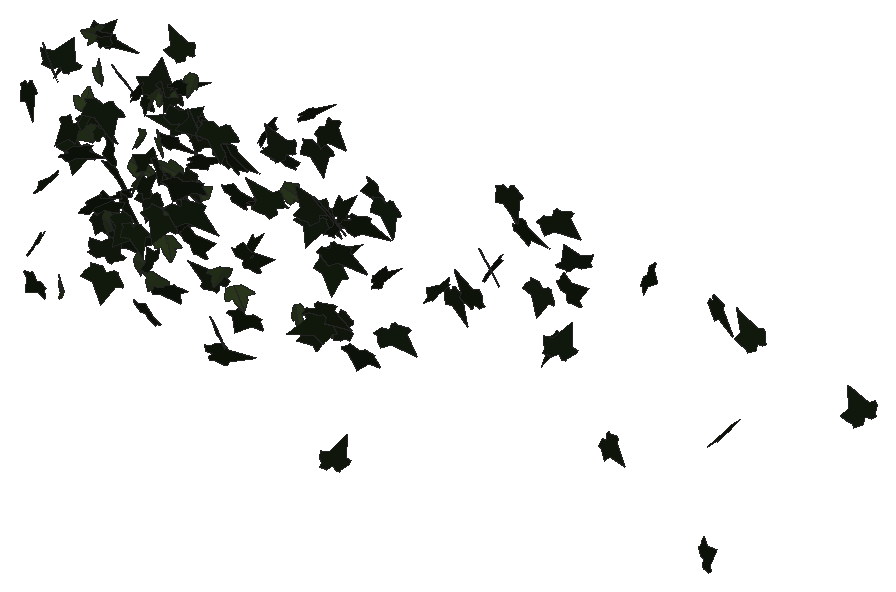
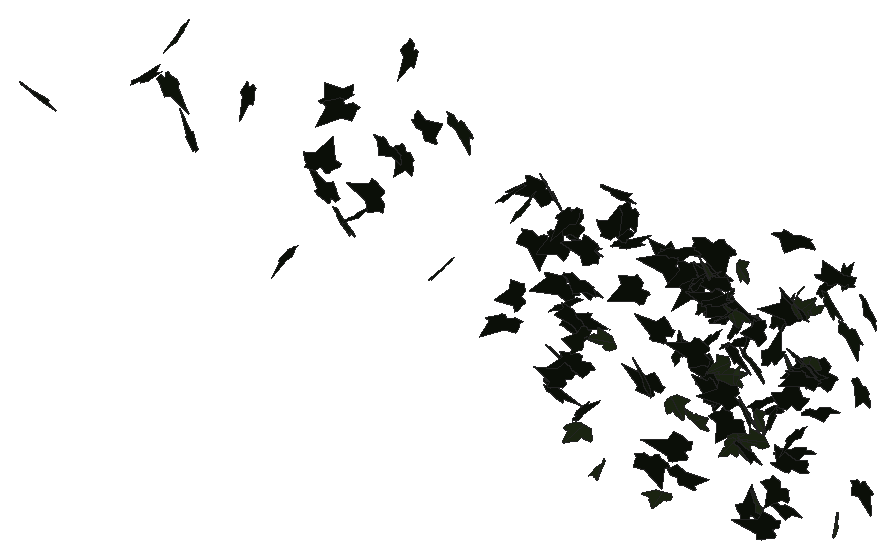
# SketchUp Ruby script. Lengths in inches.
U = 1.inch
M = Sketchup.active_model
def pt(a) = Geom::Point3d.new(a.map { |v| v * U })
def face(e, loops, mat)
  f = e.add_face(loops[0].map { |a| pt(a) })
  loops[1..].each { |l| e.add_face(l.map { |a| pt(a) }).erase! }
  f.material = f.back_material = mat if mat
  f
end
# faces: each face lists its corners as indices into pts; further lists are holes
def faces(e, pts, list, mat = nil) = list.each { |f| face(e, (f[0].is_a?(Array) ? f : [f]).map { |l| l.map { |i| pts[i] } }, mat) }
# xy, xz, yz: faces in a plane at the given z, y or x. An outline is a flat list of corners, or four numbers for a rectangle; further outlines are holes
def ring(l) = l.size == 4 ? [[l[0], l[1]], [l[2], l[1]], [l[2], l[3]], [l[0], l[3]]] : l.each_slice(2).to_a
def flat(e, list, mat, &to3) = list.each { |f| face(e, (f[0].is_a?(Array) ? f : [f]).map { |l| ring(l).map { |u, v| to3.(u, v) } }, mat) }
def xy(e, z, list, mat = nil) = flat(e, list, mat) { |x, y| [x, y, z] }
def xz(e, y, list, mat = nil) = flat(e, list, mat) { |x, z| [x, y, z] }
def yz(e, x, list, mat = nil) = flat(e, list, mat) { |y, z| [x, y, z] }
def lines(e, pts, list) = list.each { |a, b| e.add_line(pt(pts[a]), pt(pts[b])) }
# prism: a flat outline (further loops are holes) pulled along v
def prism(e, loops, v, mat = nil)
  f = face(e, loops, mat); d = Geom::Vector3d.new(v.map { |x| x * U })
  f.pushpull(f.normal.samedirection?(d) ? d.length : -d.length)
end
def box(e, o, s, mat = nil) = prism(e, [[o, [o[0] + s[0], o[1], o[2]], [o[0] + s[0], o[1] + s[1], o[2]], [o[0], o[1] + s[1], o[2]]]], [0, 0, s[2]], mat)
def at(x, y, z, deg = 0) = Geom::Transformation.translation(pt([x, y, z])) * Geom::Transformation.rotation(ORIGIN, Z_AXIS, deg.degrees)
def axes(o, x, y, z) = Geom::Transformation.new([*x, 0, *y, 0, *z, 0, *pt(o).to_a, 1])
def part(name) = M.definitions.add(name)
# library, detail: a bought-in or finely detailed component or shape, given as its bounding box
def library(name, o, s) = part(name).tap { |d| box(d.entities, o, s) }
def detail(e, o, s) = box(e.add_group.entities, o, s)
def put(e, d, t, mat = nil) = e.add_instance(d, t).tap { |i| i.material = mat if mat }
def group(e, t, mat = nil) = e.add_group.tap { |g| g.transformation = t; g.material = mat if mat }.entities
root = M.entities
M.materials.add("1026 AP 7946 SUNNY SIDE UP").color = [254, 231, 186]
M.materials.add("efeu1").color = [18, 25, 13]
M.materials.add("efeu2").color = [43, 57, 29]
c1 = part("ivyleaf_9")
p = [[1.54,2.16,1.25],[1.36,2.04,1.19],[-0.21,0.99,0.68],[-0.71,1.11,0.82],[-0.85,0.86,0.67],[-0.8,0.17,0.21],
  [-0.9,-0.01,0.1],[-0.67,-0.16,-0.02],[-0.08,-0.08,-0.05],[-0.03,-0.6,-0.4],[0.65,-0.88,-0.66],[0.83,-0.6,-0.49],
  [1.29,-0.42,-0.43],[1.8125,-0.07,-0.26],[1.21,0.44,0.15]]
faces(c1.entities,p,[[0,1,2,3,4,5,6,7,8,9,10,11,12,13,14]],"efeu1")
c2 = part("ivyleaf_10")
p = [[0,0.5,-0.03],[-0.0625,2.02,-0.43],[-0.19,2.01,-0.46],[-0.54,1.05,-0.29],[-0.52,0.625,-0.18],[-0.83,0.76,-0.28],
  [-1.16,0.64,-0.33],[-1.15,0.33,-0.24],[-0.77,-0.39,0.02],[-0.3,-0.51,0.16],[0.04,-0.48,0.23],[-0.02,2.01,-0.4375],
  [-0.06,2.01,-0.43],[0.04,-0.49,0.23],[0.67,-0.49,0.14],[1.38,0.36,-0.2],[1.375,0.51,-0.24],[0.81,0.65,-0.19],
  [0.62,0.59,-0.15],[0.6,1.09,-0.28],[0.5,1.23,-0.31]]
faces(c2.entities,p,[[0,1,2,3,4,5,6,7,8,9,10],[11,12,0,13,14,15,16,17,18,19,20]],"efeu2")
put(root,c1,axes([151.82,207.26,278],[-0.24756,-0.03572,-0.44913],[0.67689,-0.09372,-0.15286],[-0.12031,-0.45376,0.06414]),"1026 AP 7946 SUNNY SIDE UP")
put(root,c1,axes([152.5,206.9,269.13],[0.28075,-0.0031,-0.35331],[-0.53519,-0.04898,-0.18239],[-0.06608,0.38352,-0.02386]),"1026 AP 7946 SUNNY SIDE UP")
put(root,c1,axes([152.38,210,274.16],[-0.35586,-0.33275,-0.04194],[0.06626,0.0182,-0.41369],[0.52258,-0.2289,0.02389]),"1026 AP 7946 SUNNY SIDE UP")
put(root,c1,axes([152.53,209.19,279.03],[-0.43904,0.15154,-0.27988],[0.32861,-0.18058,-0.32507],[-0.36393,-0.34588,0.04413]),"1026 AP 7946 SUNNY SIDE UP")
put(root,c2,axes([152.61,210.9,279.26],[-0.12966,-0.13523,-0.37237],[-0.27517,-0.31545,0.16121],[-0.53958,0.19336,0.00727]),"1026 AP 7946 SUNNY SIDE UP")
put(root,c2,axes([152.37,208.8125,267.83],[-0.24827,0.26391,0.24196],[0.22958,-0.18372,0.31472],[0.50413,0.21364,-0.02417]),"1026 AP 7946 SUNNY SIDE UP")
put(root,c1,axes([152.98,207.5,279.03],[0.12702,-0.28237,0.28323],[-0.02585,0.27961,0.30071],[-0.62091,-0.0694,0.04542]),"1026 AP 7946 SUNNY SIDE UP")
put(root,c1,axes([152.82,211.95,271.16],[0.25313,0.30382,0.15856],[0.11657,0.13294,-0.35342],[-0.52144,0.1772,-0.00204]),"1026 AP 7946 SUNNY SIDE UP")
put(root,c1,axes([152.85,211.79,270.22],[-0.46073,-0.1525,-0.18223],[0.27103,0.04824,-0.33836],[0.24627,-0.3384,0.03146]),"1026 AP 7946 SUNNY SIDE UP")
put(root,c1,axes([152.73,210.84,279.09],[-0.25642,0.25226,0.25673],[0.24899,-0.19186,0.30748],[0.49712,0.22621,-0.02158]),"1026 AP 7946 SUNNY SIDE UP")
put(root,c1,axes([152.99,207.91,279.1875],[-0.50481,0.03533,0.30289],[0.46211,-0.01274,0.33233],[0.05453,0.435,-0.0123]),"1026 AP 7946 SUNNY SIDE UP")
put(root,c1,axes([153.37,209.45,275.3],[-0.56661,-0.00848,0.10386],[0.15663,0.03656,0.36999],[-0.02828,0.37241,-0.03175]),"1026 AP 7946 SUNNY SIDE UP")
put(root,c1,axes([152.88,210.15,275.64],[-0.03711,-0.17458,-0.36196],[0.33349,0.28932,-0.16154],[0.51735,-0.19902,0.07816]),"1026 AP 7946 SUNNY SIDE UP")
put(root,c1,axes([152.85,210.92,279.09],[0.44229,-0.01607,0.27492],[0.41238,-0.05932,-0.2887],[0.08237,0.38323,-0.03086]),"1026 AP 7946 SUNNY SIDE UP")
put(root,c1,axes([153.64,209.9,276.29],[-0.60373,0.08396,-0.11642],[0.1608,-0.0613,-0.40349],[-0.15302,-0.39565,0.03534]),"1026 AP 7946 SUNNY SIDE UP")
put(root,c2,axes([153.46,209.09,275.7],[-0.14164,-0.3356,-0.18528],[0.14848,0.15735,-0.35405],[0.57854,-0.12255,0.04551]),"1026 AP 7946 SUNNY SIDE UP")
put(root,c1,axes([153.25,208.29,274.9],[0.46661,0.23817,0.28253],[0.34831,0.1598,-0.39088],[-0.45063,0.37013,-0.00958]),"1026 AP 7946 SUNNY SIDE UP")
put(root,c1,axes([153.46,211.64,276.96],[0.45549,-0.32431,-0.05035],[0.08353,-0.01548,0.44688],[-0.50847,-0.29306,0.0283]),"1026 AP 7946 SUNNY SIDE UP")
put(root,c1,axes([153.27,212.01,269.06],[0.20685,0.07039,0.39309],[0.6001,0.04682,-0.14432],[-0.1065,0.4005,-0.04977]),"1026 AP 7946 SUNNY SIDE UP")
put(root,c1,axes([154.17,204.8125,272.35],[-0.26094,0.12894,-0.38017],[-0.3891,0.27672,0.21544],[0.47723,0.29612,-0.03222]),"1026 AP 7946 SUNNY SIDE UP")
put(root,c2,axes([154.23,208.99,278.51],[-0.02563,0.25828,-0.28808],[-0.07963,0.27741,0.26723],[0.59494,0.04825,0.02335]),"1026 AP 7946 SUNNY SIDE UP")
put(root,c2,axes([154.08,208.24,277.47],[0.28619,0.30022,-0.15927],[0.09743,0.14492,0.36193],[0.52322,-0.1912,0.01972]),"1026 AP 7946 SUNNY SIDE UP")
put(root,c1,axes([154.41,205.29,275.1875],[-0.09972,0.39838,0.14057],[-0.05291,0.13046,-0.41462],[-0.65887,-0.07077,0.01202]),"1026 AP 7946 SUNNY SIDE UP")
put(root,c2,axes([153.875,211.86,273.02],[0.16086,0.08926,0.36373],[0.5276,0.1181,-0.13042],[-0.22058,0.34759,-0.04669]),"1026 AP 7946 SUNNY SIDE UP")
put(root,c1,axes([154.29,208.92,271.96],[0.21865,-0.26612,-0.3162],[-0.22842,0.26868,-0.30774],[0.59461,0.20107,-0.00194]),"1026 AP 7946 SUNNY SIDE UP")
put(root,c1,axes([154.56,208.97,270.1875],[-0.38808,0.01838,0.32993],[0.49752,-0.0518,0.25404],[0.08207,0.40091,0.02008]),"1026 AP 7946 SUNNY SIDE UP")
put(root,c1,axes([155.29,212.125,277],[-0.06316,-0.03237,-0.39158],[-0.59942,-0.0046,0.0419],[-0.01258,0.38201,-0.03043]),"1026 AP 7946 SUNNY SIDE UP")
put(root,c2,axes([154.97,210.73,273.24],[0.16985,-0.37206,0.10825],[0.03224,-0.10563,-0.39962],[0.60797,0.10955,-0.00905]),"1026 AP 7946 SUNNY SIDE UP")
put(root,c1,axes([154.9,206.28,277.74],[0.07222,-0.09335,-0.44026],[0.34225,-0.36724,0.10472],[-0.59568,-0.22231,0.00679]),"1026 AP 7946 SUNNY SIDE UP")
put(root,c1,axes([154.9,210.53,277.27],[0.13207,0.09677,0.38571],[0.3255,0.3117,-0.12921],[-0.51261,0.22286,0.01733]),"1026 AP 7946 SUNNY SIDE UP")
put(root,c2,axes([154.74,210.9,269.12],[0.09384,-0.11595,-0.3656],[0.31918,-0.29076,0.13158],[-0.49153,-0.21095,0.01565]),"1026 AP 7946 SUNNY SIDE UP")
put(root,c1,axes([155.02,211.5,272.0625],[-0.46932,-0.04868,-0.24063],[0.3706,-0.00485,-0.30962],[0.05556,-0.3788,0.03263]),"1026 AP 7946 SUNNY SIDE UP")
put(root,c1,axes([155.0625,208.35,272.82],[0.44426,0.14474,0.25341],[-0.37328,-0.07089,0.32455],[0.24712,-0.36729,0.03466]),"1026 AP 7946 SUNNY SIDE UP")
put(root,c1,axes([155.08,209.55,272.69],[0.41381,-0.23166,-0.26365],[-0.31719,0.15591,-0.36003],[0.43859,0.33133,-0.01162]),"1026 AP 7946 SUNNY SIDE UP")
put(root,c1,axes([155.35,210.62,277.29],[0.21274,-0.13117,-0.36494],[-0.41014,0.23864,-0.19267],[0.42812,0.2938,-0.00323]),"1026 AP 7946 SUNNY SIDE UP")
put(root,c1,axes([155.3,206.95,273.74],[-0.04608,0.21893,-0.35523],[-0.09773,0.34055,0.22936],[0.63644,0.06815,0.0095]),"1026 AP 7946 SUNNY SIDE UP")
put(root,c1,axes([155.3,210.6,272.78],[-0.17761,0.30682,0.2428],[0.08346,-0.22909,0.33458],[0.60091,0.1225,0.02529]),"1026 AP 7946 SUNNY SIDE UP")
put(root,c1,axes([155.56,207.77,270.16],[-0.37992,-0.3558,-0.07561],[0.09115,0.0468,-0.44225],[0.56329,-0.24755,0.02057]),"1026 AP 7946 SUNNY SIDE UP")
put(root,c1,axes([155.35,211.96,274.64],[0.4787,-0.01417,0.24114],[0.36564,-0.03226,-0.31367],[0.04854,0.38271,-0.01526]),"1026 AP 7946 SUNNY SIDE UP")
put(root,c2,axes([156.05,210.83,274.92],[-0.06523,0.20533,-0.35456],[-0.18345,0.32606,0.21607],[0.60452,0.1211,0.02731]),"1026 AP 7946 SUNNY SIDE UP")
put(root,c1,axes([156.03,210.71,277.83],[-0.64908,0.11176,0.10903],[0.17574,0.01198,0.43875],[0.16541,0.42582,-0.0383]),"1026 AP 7946 SUNNY SIDE UP")
put(root,c1,axes([156.18,212.28,278.94],[-0.44014,-0.24747,0.09737],[0.08627,0.08245,0.38455],[-0.40832,0.28418,-0.02371]),"1026 AP 7946 SUNNY SIDE UP")
put(root,c1,axes([155.92,207.78,276],[-0.09307,-0.03981,0.48579],[-0.15793,-0.46358,-0.056],[0.72752,-0.10573,0.04999]),"1026 AP 7946 SUNNY SIDE UP")
put(root,c2,axes([155.93,211.72,275.9],[0.03503,0.08339,0.38525],[0.04065,0.37294,-0.08519],[-0.60036,0.03012,0.01671]),"1026 AP 7946 SUNNY SIDE UP")
put(root,c1,axes([156.41,209.48,274.99],[-0.18493,0.31964,0.23751],[-0.15881,0.20616,-0.34909],[-0.59728,-0.15378,0.01928]),"1026 AP 7946 SUNNY SIDE UP")
put(root,c1,axes([156.1,208.76,272.28],[-0.32797,-0.33694,0.19006],[-0.11144,-0.17478,-0.40819],[0.59513,-0.21841,0.0283]),"1026 AP 7946 SUNNY SIDE UP")
put(root,c2,axes([156.04,211.04,271.72],[-0.09174,-0.1725,-0.34669],[0.21892,0.30574,-0.18506],[0.55139,-0.15009,0.01579]),"1026 AP 7946 SUNNY SIDE UP")
put(root,c2,axes([156.1,210.89,277.94],[0.63057,-0.0019,0.02835],[0.04284,-0.03648,-0.41165],[0.00689,0.40031,-0.03502]),"1026 AP 7946 SUNNY SIDE UP")
put(root,c1,axes([156.23,209.6,267.69],[0.52619,-0.20979,-0.0004],[0.03965,0.04172,0.40402],[-0.32749,-0.33203,0.04827]),"1026 AP 7946 SUNNY SIDE UP")
put(root,c2,axes([156.35,209.22,276.36],[0.06541,-0.04467,0.38865],[0.20083,-0.35605,-0.05998],[0.56299,0.1322,-0.02376]),"1026 AP 7946 SUNNY SIDE UP")
put(root,c1,axes([156.4375,211.17,277.75],[-0.17186,-0.33419,0.18321],[-0.05649,-0.17709,-0.36276],[0.59399,-0.11353,0.01851]),"1026 AP 7946 SUNNY SIDE UP")
put(root,c2,axes([156.29,206.87,273.43],[-0.01274,-0.02342,-0.40847],[0.28348,-0.35345,0.01565],[-0.55627,-0.17958,0.01733]),"1026 AP 7946 SUNNY SIDE UP")
put(root,c2,axes([157.14,210.42,274.4375],[-0.19197,-0.0504,-0.39202],[-0.6001,-0.02395,0.12937],[-0.06032,0.39864,-0.03941]),"1026 AP 7946 SUNNY SIDE UP")
put(root,c1,axes([156.72,207.125,275.58],[0.3473,-0.40408,-0.0235],[0.0654,-0.00058,0.47293],[-0.63282,-0.22182,0.03598]),"1026 AP 7946 SUNNY SIDE UP")
put(root,c1,axes([156.61,208.375,272.42],[-0.02606,-0.35621,-0.11273],[0.00879,0.10725,-0.36673],[0.58494,-0.01748,0.00049]),"1026 AP 7946 SUNNY SIDE UP")
put(root,c1,axes([156.7,206.16,279.28],[-0.36562,-0.25645,-0.29066],[0.3293,0.18821,-0.35478],[0.49896,-0.31213,0.02116]),"1026 AP 7946 SUNNY SIDE UP")
put(root,c2,axes([157.34,211.88,272.74],[0.47134,0.01451,0.25493],[-0.38748,0.05834,0.30443],[-0.04104,-0.38425,0.05355]),"1026 AP 7946 SUNNY SIDE UP")
put(root,c1,axes([156.75,210.91,278.1],[0.26049,0.29605,-0.22411],[0.11465,0.20926,0.34912],[0.56778,-0.17808,0.03232]),"1026 AP 7946 SUNNY SIDE UP")
put(root,c2,axes([157.24,209.05,278.85],[0.08869,-0.344,0.14593],[0.0348,-0.1419,-0.35994],[0.58511,0.06058,-0.00071]),"1026 AP 7946 SUNNY SIDE UP")
put(root,c1,axes([157.62,210.34,276.92],[-0.24354,-0.00817,0.38364],[-0.54881,-0.13781,-0.15345],[0.20476,-0.37909,0.04501]),"1026 AP 7946 SUNNY SIDE UP")
put(root,c2,axes([157.69,208.61,270.31],[-0.55614,-0.05787,0.18526],[-0.26817,-0.06793,-0.36781],[0.12888,-0.39107,0.03407]),"1026 AP 7946 SUNNY SIDE UP")
put(root,c1,axes([157.87,207.99,271.4375],[-0.32059,0.08095,-0.33422],[-0.43237,0.17655,0.22412],[0.30038,0.34052,-0.03411]),"1026 AP 7946 SUNNY SIDE UP")
put(root,c1,axes([157.79,208.72,275.47],[-0.05047,-0.22248,0.35576],[0.00399,-0.34775,-0.23175],[0.6476,-0.01519,0.02915]),"1026 AP 7946 SUNNY SIDE UP")
put(root,c1,axes([158.21,209.16,273.08],[0.43539,0.2904,-0.11337],[-0.08783,-0.10069,-0.41294],[-0.48129,0.28108,-0.0272]),"1026 AP 7946 SUNNY SIDE UP")
put(root,c2,axes([158.18,210.32,279.28],[0.45128,-0.2577,0.06672],[0.04899,-0.06419,-0.3968],[0.41549,0.28746,-0.02568]),"1026 AP 7946 SUNNY SIDE UP")
put(root,c1,axes([157.78,210.18,273.16],[0.33761,-0.11013,-0.33392],[0.5354,0.0364,0.22025],[-0.04576,-0.38656,0.1134]),"1026 AP 7946 SUNNY SIDE UP")
put(root,c1,axes([158.72,211.26,269.26],[-0.06373,0.05576,0.39552],[-0.52464,0.19134,-0.06385],[-0.31031,-0.33495,0.02671]),"1026 AP 7946 SUNNY SIDE UP")
put(root,c1,axes([158.05,210.58,275.16],[0.24414,0.27587,-0.26124],[0.16394,0.23361,0.32693],[0.56767,-0.18611,0.01794]),"1026 AP 7946 SUNNY SIDE UP")
put(root,c1,axes([158.49,209.92,276.79],[0.30154,-0.35884,-0.00227],[0.0414,0.01388,0.41811],[-0.56272,-0.19127,0.02954]),"1026 AP 7946 SUNNY SIDE UP")
put(root,c1,axes([158.32,209.27,277.68],[-0.27526,0.0767,0.36469],[0.52714,-0.11327,0.19565],[0.21386,0.37792,-0.01287]),"1026 AP 7946 SUNNY SIDE UP")
put(root,c1,axes([158.55,209.34,275.21],[0.21791,-0.33602,-0.26542],[-0.18491,0.22779,-0.37267],[0.63771,0.18087,-0.01736]),"1026 AP 7946 SUNNY SIDE UP")
put(root,c1,axes([158.67,207.79,270.54],[0.47819,0.25131,0.0017],[0.02969,-0.02249,-0.40543],[-0.39404,0.30328,-0.02848]),"1026 AP 7946 SUNNY SIDE UP")
put(root,c1,axes([158.79,207.57,274.11],[-0.29602,-0.38942,0.11959],[-0.04038,-0.11872,-0.44539],[0.63868,-0.188,0.02727]),"1026 AP 7946 SUNNY SIDE UP")
put(root,c2,axes([158.61,207.99,272.72],[0.56617,0.00438,0.16453],[0.25063,-0.03576,-0.36947],[0.01653,0.39226,-0.03321]),"1026 AP 7946 SUNNY SIDE UP")
put(root,c1,axes([159.15,209.63,277.74],[-0.23625,-0.15329,0.36906],[-0.31543,-0.29981,-0.22006],[0.52674,-0.24829,0.03375]),"1026 AP 7946 SUNNY SIDE UP")
put(root,c1,axes([158.76,207.98,275.69],[0.21101,-0.28323,0.31093],[0.16298,-0.28592,-0.32385],[0.63199,0.1683,-0.0203]),"1026 AP 7946 SUNNY SIDE UP")
put(root,c2,axes([159.07,212.0625,268.7],[0.3811,0.29446,0.10292],[0.13407,0.05668,-0.39143],[-0.46932,0.2553,-0.02825]),"1026 AP 7946 SUNNY SIDE UP")
put(root,c1,axes([159.3125,209.48,277.46],[0.08078,-0.12222,-0.45729],[-0.21282,0.42217,-0.13363],[0.69086,0.14434,0.01231]),"1026 AP 7946 SUNNY SIDE UP")
put(root,c1,axes([159.27,207.69,275.89],[0.09829,-0.41756,0.164],[0.04849,-0.15873,-0.43584],[0.70234,0.06939,0.00714]),"1026 AP 7946 SUNNY SIDE UP")
put(root,c1,axes([159.32,209.53,278],[0.63422,-0.09811,0.05207],[0.06379,-0.04853,-0.42619],[0.16181,0.40366,-0.03605]),"1026 AP 7946 SUNNY SIDE UP")
put(root,c1,axes([159.73,208.3125,272.81],[-0.02922,0.01266,0.46345],[0.44296,-0.35071,0.02011],[0.55172,0.28224,0.0084]),"1026 AP 7946 SUNNY SIDE UP")
put(root,c2,axes([160.58,209.32,271.39],[-0.22149,-0.34264,0.13665],[-0.06158,-0.12935,-0.3822],[0.57556,-0.1457,0.01169]),"1026 AP 7946 SUNNY SIDE UP")
put(root,c1,axes([160.71,208.875,278.4],[-0.29864,-0.39101,-0.14525],[0.10946,0.12043,-0.44701],[0.64315,-0.20205,0.00863]),"1026 AP 7946 SUNNY SIDE UP")
put(root,c1,axes([161.02,210.3125,268.94],[0.32803,0.14975,-0.30826],[-0.33366,-0.21472,-0.26362],[-0.40835,0.29574,-0.03223]),"1026 AP 7946 SUNNY SIDE UP")
put(root,c1,axes([161.14,206.01,277.25],[0.35413,0.30106,-0.30736],[-0.26558,-0.24824,-0.38863],[-0.61333,0.28132,-0.00919]),"1026 AP 7946 SUNNY SIDE UP")
put(root,c1,axes([160.7,209.84,274.79],[0.15823,-0.0691,0.38755],[0.46623,-0.23227,-0.12689],[0.38087,0.31303,-0.00567]),"1026 AP 7946 SUNNY SIDE UP")
put(root,c1,axes([161.05,206.06,276],[-0.0167,-0.13825,-0.47593],[0.39392,0.39236,-0.12482],[0.64652,-0.24264,0.06376]),"1026 AP 7946 SUNNY SIDE UP")
put(root,c1,axes([161.29,210.16,272.2],[-0.04051,0.32703,0.26643],[0.02475,-0.25631,0.33643],[0.65332,0.02999,0.00378]),"1026 AP 7946 SUNNY SIDE UP")
put(root,c1,axes([160.99,208.8,277.53],[0.19758,-0.00471,-0.44974],[0.61161,0.20745,0.11425],[0.31166,-0.40412,0.0609]),"1026 AP 7946 SUNNY SIDE UP")
put(root,c1,axes([161.24,207.96,268.24],[0.28831,0.02439,0.39076],[0.59734,-0.00436,-0.18899],[-0.01051,0.42115,-0.02211]),"1026 AP 7946 SUNNY SIDE UP")
put(root,c1,axes([161.33,209.83,271.98],[0.03854,0.01679,0.42314],[0.52102,-0.24417,-0.01151],[0.3823,0.33107,-0.02696]),"1026 AP 7946 SUNNY SIDE UP")
put(root,c1,axes([161.44,208.56,277.47],[0.17919,-0.14588,0.42432],[0.29146,-0.37027,-0.18972],[0.62355,0.21499,-0.03326]),"1026 AP 7946 SUNNY SIDE UP")
put(root,c2,axes([162.33,212.0625,268.92],[0.00643,0.39618,-0.07263],[-0.00528,-0.07272,-0.40858],[-0.63335,0.00463,0.00267]),"1026 AP 7946 SUNNY SIDE UP")
put(root,c2,axes([162.18,211.67,274.76],[0.17287,0.04656,0.39341],[0.58124,0.09627,-0.12125],[-0.16612,0.3853,-0.01482]),"1026 AP 7946 SUNNY SIDE UP")
put(root,c1,axes([162.85,208.79,275.79],[0.44505,0.20435,0.22825],[0.31551,0.09693,-0.35747],[-0.35186,0.34539,-0.03184]),"1026 AP 7946 SUNNY SIDE UP")
put(root,c1,axes([163.34,208.76,279.3],[-0.09947,0.04789,-0.4684],[-0.43066,0.36389,0.08083],[0.57613,0.28028,-0.02045]),"1026 AP 7946 SUNNY SIDE UP")
put(root,c1,axes([163.12,211.59,278.74],[0.09005,0.3393,-0.21385],[0.0227,0.20976,0.35525],[0.62663,-0.05636,0.01786]),"1026 AP 7946 SUNNY SIDE UP")
put(root,c1,axes([163.17,205.65,271.12],[0.36555,-0.23805,-0.25762],[0.371,-0.10839,0.33344],[-0.39424,-0.32273,0.07491]),"1026 AP 7946 SUNNY SIDE UP")
put(root,c1,axes([163.55,211.9,277.27],[-0.37486,-0.1296,-0.31205],[0.45118,0.10024,-0.27692],[0.25244,-0.37161,0.03154]),"1026 AP 7946 SUNNY SIDE UP")
put(root,c1,axes([163.5,211.8,274.36],[0.34536,-0.34525,0.16597],[0.11972,-0.14474,-0.4222],[0.58832,0.23212,-0.01151]),"1026 AP 7946 SUNNY SIDE UP")
put(root,c1,axes([163.95,208.94,278.05],[0.57648,-0.09747,0.17484],[-0.23327,0.09844,0.3877],[-0.20189,-0.39206,0.05129]),"1026 AP 7946 SUNNY SIDE UP")
put(root,c1,axes([164.7,207.6,276.6875],[-0.44683,-0.32746,-0.00849],[-0.03957,0.01341,0.44582],[-0.51347,0.28393,-0.02697]),"1026 AP 7946 SUNNY SIDE UP")
put(root,c2,axes([164.34,210.87,269.48],[-0.36141,-0.2171,-0.26054],[0.32876,0.14342,-0.32333],[0.40626,-0.30919,0.02987]),"1026 AP 7946 SUNNY SIDE UP")
put(root,c1,axes([165.01,207.89,279.24],[-0.6145,-0.05121,-0.11951],[-0.18804,0.02672,0.40407],[-0.06502,0.4067,-0.03917]),"1026 AP 7946 SUNNY SIDE UP")
put(root,c1,axes([164.46,211.83,272.23],[-0.02854,0.01471,0.41957],[0.58842,0.16183,0.01211],[-0.25343,0.37409,-0.01913]),"1026 AP 7946 SUNNY SIDE UP")
put(root,c1,axes([164.48,211.05,274.85],[-0.03648,-0.10129,-0.40569],[0.62398,0.07785,-0.04432],[0.13537,-0.38614,0.09497]),"1026 AP 7946 SUNNY SIDE UP")
put(root,c1,axes([165.1,210.04,269.54],[-0.16538,-0.13728,0.37754],[-0.30602,-0.3118,-0.17932],[0.53518,-0.22072,0.01413]),"1026 AP 7946 SUNNY SIDE UP")
put(root,c1,axes([165.18,210.48,279.32],[0.1209,-0.22163,-0.41956],[-0.24955,0.37395,-0.23907],[0.68318,0.17582,-0.01308]),"1026 AP 7946 SUNNY SIDE UP")
put(root,c1,axes([165.39,209.52,275.42],[-0.54589,-0.12578,-0.17791],[0.27954,0.01025,-0.37735],[0.18467,-0.3873,0.04529]),"1026 AP 7946 SUNNY SIDE UP")
put(root,c1,axes([166.37,208.4,276.5625],[-0.6277,-0.04291,-0.1843],[-0.28572,0.02897,0.41129],[-0.04276,0.43639,-0.04284]),"1026 AP 7946 SUNNY SIDE UP")
put(root,c1,axes([166.5,210.17,270.41],[-0.31602,-0.07147,-0.37746],[-0.56591,-0.07165,0.2176],[-0.15348,0.41135,-0.02512]),"1026 AP 7946 SUNNY SIDE UP")
put(root,c1,axes([165.77,209.12,271.43],[0.04473,-0.06159,-0.42876],[0.3218,0.36609,-0.03929],[0.57738,-0.19927,0.05512]),"1026 AP 7946 SUNNY SIDE UP")
put(root,c1,axes([166.62,209.09,273.86],[-0.15662,-0.41253,0.02185],[0.00688,-0.02528,-0.43722],[0.64968,-0.09918,0.0099]),"1026 AP 7946 SUNNY SIDE UP")
put(root,c1,axes([166.62,208.16,277.27],[0.61353,-0.25096,0.03782],[0.01821,-0.05226,-0.47667],[0.39872,0.38855,-0.03643]),"1026 AP 7946 SUNNY SIDE UP")
put(root,c1,axes([167.44,207.4,272.09],[-0.02046,-0.09351,-0.435],[-0.1551,-0.41013,0.09442],[-0.66128,0.09908,-0.00868]),"1026 AP 7946 SUNNY SIDE UP")
put(root,c1,axes([166.71,208.96,274.71],[-0.00352,-0.04022,-0.4522],[0.45301,0.33178,-0.03091],[0.52408,-0.28705,0.02367]),"1026 AP 7946 SUNNY SIDE UP")
put(root,c1,axes([167.3125,208.38,276.32],[-0.08078,0.17362,-0.39719],[-0.14938,0.37474,0.1886],[0.64932,0.10781,-0.00602]),"1026 AP 7946 SUNNY SIDE UP")
put(root,c1,axes([168.08,207.65,277.45],[-0.12912,0.32535,0.29742],[0.13343,-0.27426,0.34387],[0.66885,0.11752,-0.01118]),"1026 AP 7946 SUNNY SIDE UP")
put(root,c1,axes([168.5,209.73,277.76],[0.26454,-0.34928,-0.20028],[0.17971,-0.15786,0.3972],[-0.60074,-0.20103,0.03063]),"1026 AP 7946 SUNNY SIDE UP")
put(root,c1,axes([168.67,209.45,273.67],[0.13097,0.15282,0.40724],[0.39738,0.3044,-0.17469],[-0.53338,0.26431,-0.03016]),"1026 AP 7946 SUNNY SIDE UP")
put(root,c1,axes([169.19,207.27,277.67],[0.07618,0.02885,-0.43052],[0.40081,0.33201,0.05598],[0.52301,-0.25864,0.01981]),"1026 AP 7946 SUNNY SIDE UP")
put(root,c1,axes([169.7,208.79,277.96],[0.03284,-0.44898,-0.01368],[-0.01153,0.01039,-0.46292],[0.70608,0.02105,-0.00692]),"1026 AP 7946 SUNNY SIDE UP")
put(root,c1,axes([169.83,208.96,271.92],[-0.01654,-0.21455,-0.38634],[0.13282,0.36563,-0.21651],[0.66455,-0.07842,0.03366]),"1026 AP 7946 SUNNY SIDE UP")
put(root,c1,axes([170.43,204.39,267.75],[-0.51943,0.30906,0.0587],[0.0958,-0.01554,0.46491],[0.48428,0.33457,-0.02901]),"1026 AP 7946 SUNNY SIDE UP")
put(root,c1,axes([171.53,204.74,273.375],[0.49421,0.1323,-0.28109],[-0.36918,-0.14421,-0.35054],[-0.30342,0.39095,-0.03132]),"1026 AP 7946 SUNNY SIDE UP")
put(root,c1,axes([172.22,210.1,274.09],[0.25678,-0.41251,-0.06363],[-0.06247,0.04812,-0.45635],[0.65234,0.16699,-0.01865]),"1026 AP 7946 SUNNY SIDE UP")
put(root,c1,axes([174.5625,210.89,279.42],[-0.30644,-0.08863,-0.38755],[0.59342,0.04461,-0.21227],[0.12744,-0.42087,0.05652]),"1026 AP 7946 SUNNY SIDE UP")
put(root,c1,axes([174.45,211.71,277.38],[0.3087,-0.00339,-0.43944],[0.66546,0.06024,0.20053],[0.08384,-0.46567,0.02637]),"1026 AP 7946 SUNNY SIDE UP")
put(root,c1,axes([175.58,204.93,277.53],[-0.12808,0.42293,0.19018],[-0.10743,0.17188,-0.44148],[-0.71609,-0.10143,0.03222]),"1026 AP 7946 SUNNY SIDE UP")
put(root,c1,axes([175.86,208.16,277.38],[-0.18094,0.11893,-0.44882],[-0.41361,0.34865,0.17141],[0.57847,0.28649,-0.01783]),"1026 AP 7946 SUNNY SIDE UP")
put(root,c1,axes([176.79,205.78,277.13],[0.11828,-0.07886,0.43918],[-0.35187,0.36405,0.11207],[-0.58467,-0.23505,0.0214]),"1026 AP 7946 SUNNY SIDE UP")
put(root,c1,axes([176.42,210.79,275.41],[-0.13601,-0.40631,0.13163],[-0.03251,-0.12857,-0.42866],[0.67004,-0.08872,0.00592]),"1026 AP 7946 SUNNY SIDE UP")
put(root,c1,axes([177.83,209.83,279.76],[-0.02359,-0.14794,-0.45261],[0.00274,0.43871,-0.14997],[0.72768,-0.00645,-0.01411]),"1026 AP 7946 SUNNY SIDE UP")
put(root,c1,axes([178.2,210.81,277.17],[0.38078,0.1329,0.35208],[-0.50918,-0.11275,0.28151],[0.26819,-0.40277,0.03457]),"1026 AP 7946 SUNNY SIDE UP")
put(root,c1,axes([178.27,209.57,274.1875],[-0.50585,0.11688,-0.2816],[0.3631,-0.15695,-0.34918],[-0.29593,-0.39236,0.05293]),"1026 AP 7946 SUNNY SIDE UP")
put(root,c1,axes([178.12,204.88,280.05],[0.55764,-0.18757,-0.26042],[-0.38244,0.07592,-0.41086],[0.31207,0.42822,-0.03816]),"1026 AP 7946 SUNNY SIDE UP")
put(root,c1,axes([177.88,210.71,275.8],[-0.06632,0.07719,0.44324],[0.37368,-0.35821,0.0882],[0.57606,0.24125,-0.00618]),"1026 AP 7946 SUNNY SIDE UP")
put(root,c1,axes([181.64,208.6875,270.89],[0.24419,-0.27197,-0.33054],[-0.2717,0.26877,-0.32084],[0.60095,0.23203,-0.01075]),"1026 AP 7946 SUNNY SIDE UP")
put(root,c1,axes([181.76,205.26,276.72],[-0.35569,-0.09077,0.3912],[0.49268,0.22063,0.24757],[-0.36761,0.38352,-0.04672]),"1026 AP 7946 SUNNY SIDE UP")
put(root,c1,axes([182.83,209.875,278.76],[0.044,-0.08579,-0.4689],[-0.48154,0.33802,-0.08314],[0.54539,0.30537,-0.03558]),"1026 AP 7946 SUNNY SIDE UP")
put(root,c1,axes([187.32,208.72,279.49],[0.40683,-0.35334,-0.19773],[-0.21394,0.13531,-0.44948],[0.59337,0.29104,-0.0265]),"1026 AP 7946 SUNNY SIDE UP")
put(root,c1,axes([188.37,210.13,277.39],[-0.38288,-0.35272,0.17526],[0.1185,0.15678,0.44171],[-0.60566,0.25366,-0.02438]),"1026 AP 7946 SUNNY SIDE UP")
put(root,c1,axes([189.85,206.57,275.29],[-0.35514,0.37387,-0.16258],[0.09949,-0.14842,-0.45032],[-0.63162,-0.23359,0.02049]),"1026 AP 7946 SUNNY SIDE UP")
put(root,c1,axes([190.75,203.74,270.68],[-0.03364,0.16493,0.45425],[0.12794,-0.4325,0.16856],[0.72771,0.08366,-0.00864]),"1026 AP 7946 SUNNY SIDE UP")
put(root,c1,axes([193.54,210.92,275.32],[-0.6694,0.06028,-0.21842],[-0.31633,0.08394,0.44052],[0.14287,0.46828,-0.04798]),"1026 AP 7946 SUNNY SIDE UP")
